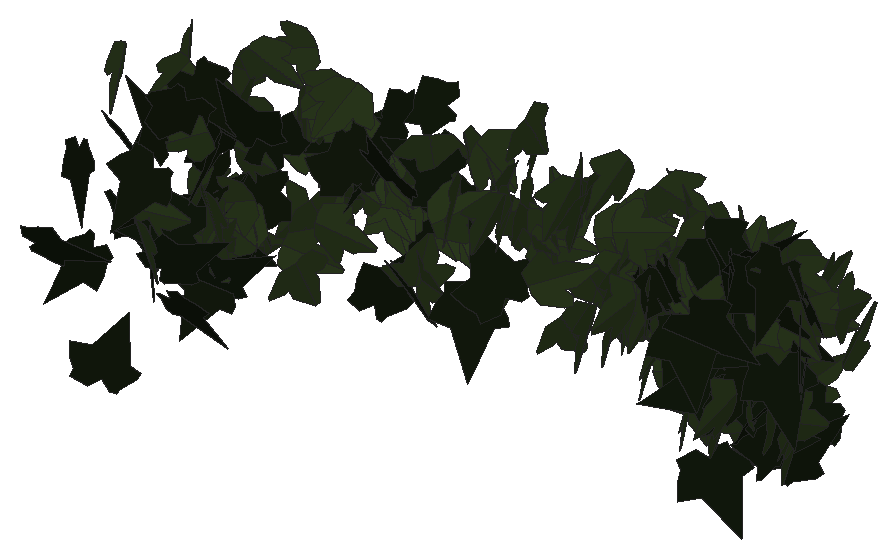
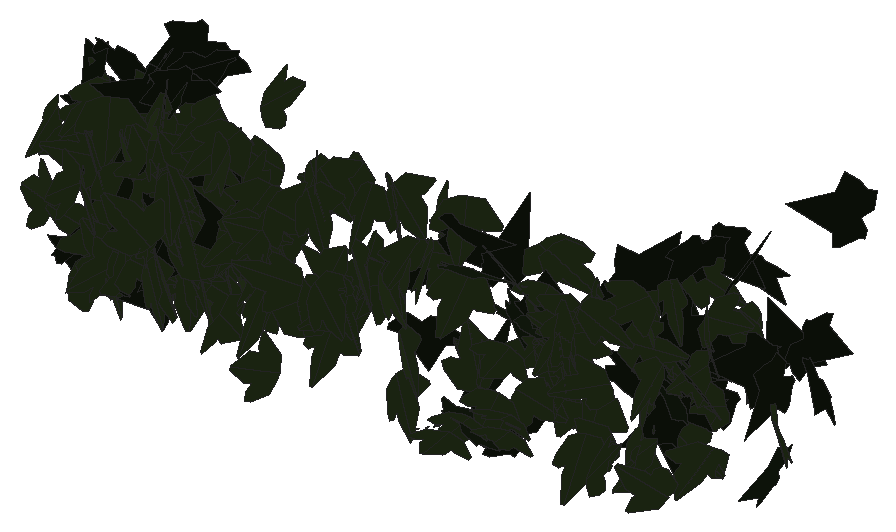
# SketchUp Ruby script. Lengths in inches.
U = 1.inch
M = Sketchup.active_model
def pt(a) = Geom::Point3d.new(a.map { |v| v * U })
def face(e, loops, mat)
  f = e.add_face(loops[0].map { |a| pt(a) })
  loops[1..].each { |l| e.add_face(l.map { |a| pt(a) }).erase! }
  f.material = f.back_material = mat if mat
  f
end
# faces: each face lists its corners as indices into pts; further lists are holes
def faces(e, pts, list, mat = nil) = list.each { |f| face(e, (f[0].is_a?(Array) ? f : [f]).map { |l| l.map { |i| pts[i] } }, mat) }
# xy, xz, yz: faces in a plane at the given z, y or x. An outline is a flat list of corners, or four numbers for a rectangle; further outlines are holes
def ring(l) = l.size == 4 ? [[l[0], l[1]], [l[2], l[1]], [l[2], l[3]], [l[0], l[3]]] : l.each_slice(2).to_a
def flat(e, list, mat, &to3) = list.each { |f| face(e, (f[0].is_a?(Array) ? f : [f]).map { |l| ring(l).map { |u, v| to3.(u, v) } }, mat) }
def xy(e, z, list, mat = nil) = flat(e, list, mat) { |x, y| [x, y, z] }
def xz(e, y, list, mat = nil) = flat(e, list, mat) { |x, z| [x, y, z] }
def yz(e, x, list, mat = nil) = flat(e, list, mat) { |y, z| [x, y, z] }
def lines(e, pts, list) = list.each { |a, b| e.add_line(pt(pts[a]), pt(pts[b])) }
# prism: a flat outline (further loops are holes) pulled along v
def prism(e, loops, v, mat = nil)
  f = face(e, loops, mat); d = Geom::Vector3d.new(v.map { |x| x * U })
  f.pushpull(f.normal.samedirection?(d) ? d.length : -d.length)
end
def box(e, o, s, mat = nil) = prism(e, [[o, [o[0] + s[0], o[1], o[2]], [o[0] + s[0], o[1] + s[1], o[2]], [o[0], o[1] + s[1], o[2]]]], [0, 0, s[2]], mat)
def at(x, y, z, deg = 0) = Geom::Transformation.translation(pt([x, y, z])) * Geom::Transformation.rotation(ORIGIN, Z_AXIS, deg.degrees)
def axes(o, x, y, z) = Geom::Transformation.new([*x, 0, *y, 0, *z, 0, *pt(o).to_a, 1])
def part(name) = M.definitions.add(name)
# library, detail: a bought-in or finely detailed component or shape, given as its bounding box
def library(name, o, s) = part(name).tap { |d| box(d.entities, o, s) }
def detail(e, o, s) = box(e.add_group.entities, o, s)
def put(e, d, t, mat = nil) = e.add_instance(d, t).tap { |i| i.material = mat if mat }
def group(e, t, mat = nil) = e.add_group.tap { |g| g.transformation = t; g.material = mat if mat }.entities
root = M.entities
M.materials.add("efeu1").color = [18, 25, 13]
M.materials.add("efeu2").color = [43, 57, 29]
c1 = part("ivyleaf_10")
p = [[0,0.5,-0.03],[-0.0625,2.02,-0.43],[-0.19,2.01,-0.46],[-0.54,1.05,-0.29],[-0.52,0.625,-0.18],[-0.83,0.76,-0.28],
  [-1.16,0.64,-0.33],[-1.15,0.33,-0.24],[-0.77,-0.39,0.02],[-0.3,-0.51,0.16],[0.04,-0.48,0.23],[-0.02,2.01,-0.4375],
  [-0.06,2.01,-0.43],[0.04,-0.49,0.23],[0.67,-0.49,0.14],[1.38,0.36,-0.2],[1.375,0.51,-0.24],[0.81,0.65,-0.19],
  [0.62,0.59,-0.15],[0.6,1.09,-0.28],[0.5,1.23,-0.31]]
faces(c1.entities,p,[[0,1,2,3,4,5,6,7,8,9,10],[11,12,0,13,14,15,16,17,18,19,20]],"efeu2")
c2 = part("ivyleaf_9")
p = [[1.54,2.16,1.25],[1.36,2.04,1.19],[-0.21,0.99,0.68],[-0.71,1.11,0.82],[-0.85,0.86,0.67],[-0.8,0.17,0.21],
  [-0.9,-0.01,0.1],[-0.67,-0.16,-0.02],[-0.08,-0.08,-0.05],[-0.03,-0.6,-0.4],[0.65,-0.88,-0.66],[0.83,-0.6,-0.49],
  [1.29,-0.42,-0.43],[1.8125,-0.07,-0.26],[1.21,0.44,0.15]]
faces(c2.entities,p,[[0,1,2,3,4,5,6,7,8,9,10,11,12,13,14]],"efeu1")
put(root,c1,axes([4.54,225.17,200.76],[0.36183,-0.29812,0.1738],[0.13554,-0.10881,-0.46882],[0.31735,0.38638,0.00207]))
put(root,c2,axes([5.6,222.72,200.27],[-0.24673,-0.00364,-0.38497],[0.39976,0.00318,-0.23762],[0.00499,-0.43497,0.00149]))
put(root,c2,axes([5.83,223.46,200.53],[0.43405,-0.05514,-0.16333],[-0.16537,0.03848,-0.42155],[0.07049,0.42977,0.01679]))
put(root,c2,axes([5.71,223.76,198.8125],[0.31945,-0.31871,0.01317],[0.01265,-0.0064,-0.45219],[0.34425,0.29599,0.0044]))
put(root,c1,axes([6.26,224.97,201.79],[0.26337,-0.21685,0.36553],[0.28954,-0.22325,-0.34106],[0.31112,0.39133,0.00798]))
put(root,c1,axes([6.8,224.12,201.73],[0.12917,0.19852,-0.38284],[-0.20895,-0.31318,-0.24103],[-0.40046,0.22745,0.00227]))
put(root,c1,axes([6.96,225.62,201.15],[-0.00251,0.23333,0.3818],[-0.1357,0.35112,-0.23291],[-0.44977,-0.10723,0.06814]))
put(root,c1,axes([7.12,223.98,198.74],[0.22464,0.36802,0.25317],[0.13154,0.21632,-0.43117],[-0.42689,0.26032,0.00037]))
put(root,c2,axes([7.32,220.92,199.6875],[-0.01481,-0.00344,-0.45216],[0.17246,-0.40463,-0.00191],[-0.43675,-0.15965,0.01458]))
put(root,c2,axes([7.18,222.16,199.75],[0.03567,0.31059,-0.31488],[-0.00014,0.30365,0.32394],[0.46844,-0.02356,0.02407]))
put(root,c1,axes([7.15,225.28,198.59],[0.23345,0.1331,-0.36738],[0.3326,0.17324,0.26387],[0.23577,-0.37616,-0.00847]))
put(root,c1,axes([7.77,223.61,198.62],[0.16189,-0.03722,-0.42292],[-0.3979,0.17451,-0.15785],[0.19022,0.39672,0.02975]))
put(root,c2,axes([7.67,222.5,201.38],[-0.03385,-0.40787,0.15384],[0.01139,0.14755,0.42544],[-0.46844,0.03306,-0.00077]))
put(root,c1,axes([7.85,224.05,201.81],[-0.37286,0.13555,0.23637],[-0.25083,0.02389,-0.38172],[-0.137,-0.41265,0.05555]))
put(root,c1,axes([7.69,223.375,200.01],[-0.01212,-0.03609,-0.45069],[0.13019,0.41625,-0.03929],[0.45124,-0.12106,-0.00077]))
put(root,c1,axes([8.11,224.7,201.01],[0.12938,0.06125,-0.43021],[-0.41855,-0.14541,-0.13912],[-0.16968,0.40538,0.01511]))
put(root,c2,axes([8.09,223.59,200.21],[-0.40829,0.21371,-0.02618],[0.02328,-0.01302,-0.45164],[-0.23123,-0.37866,0.00075]))
put(root,c2,axes([8.03,222.65,202.16],[0.03166,0.1171,-0.43463],[-0.07798,-0.41171,-0.12524],[-0.4622,0.07749,-0.00864]))
put(root,c1,axes([8.1875,222.82,201.5],[-0.18755,-0.05401,0.41096],[-0.35248,-0.22848,-0.18165],[0.24758,-0.3662,0.05272]))
put(root,c2,axes([7.87,223.53,201.07],[-0.01659,0.09814,-0.48999],[-0.16945,0.46011,0.09789],[0.47012,0.16931,0.01799]))
put(root,c1,axes([8.1875,224.66,198.61],[-0.26568,0.1929,-0.31458],[-0.27339,0.16657,0.32458],[0.27457,0.35252,0.01878]))
put(root,c2,axes([7.7,222.06,199.6875],[-0.06312,0.0246,-0.44757],[0.44742,-0.11679,-0.06546],[-0.12863,-0.41831,-0.00804]))
put(root,c1,axes([8.25,225.77,201.98],[0.19275,-0.05155,-0.40907],[-0.41552,0.08262,-0.19282],[0.10441,0.42396,-0.01216]))
put(root,c2,axes([8.27,222.5,199.64],[-0.19769,-0.07633,0.40265],[-0.3878,-0.14479,-0.20624],[0.17675,-0.40303,-0.00216]))
put(root,c2,axes([8.11,221.61,201.27],[-0.42989,-0.1683,-0.0516],[0.04917,0.01972,-0.44945],[0.18301,-0.40064,-0.00044]))
put(root,c1,axes([7.64,222.0625,200.12],[0.02616,-0.01223,-0.45152],[0.46101,-0.07957,0.0271],[-0.08656,-0.42749,0.00787]))
put(root,c2,axes([7.875,223.16,202.37],[0.06304,-0.27853,-0.34215],[-0.02745,0.32919,-0.29454],[0.46474,0.05723,0.02902]))
put(root,c1,axes([7.98,224.52,201.58],[0.20664,-0.34128,0.19772],[0.10219,-0.16491,-0.4069],[0.40935,0.21344,0.00177]))
put(root,c1,axes([8.01,221.49,200.04],[-0.32999,0.27319,-0.15156],[0.114,-0.10057,-0.42623],[-0.31437,-0.32323,0.00452]))
put(root,c2,axes([8.07,223.64,199.52],[-0.18935,0.3981,-0.00095],[-0.01202,-0.00391,0.45223],[0.42979,0.17528,0.01223]))
put(root,c1,axes([8.07,224.41,198.49],[-0.05405,-0.13447,-0.42708],[0.14284,0.38879,-0.14917],[0.44428,-0.14136,-0.004]))
put(root,c1,axes([7.88,224.97,202.06],[-0.27448,-0.04326,-0.36439],[0.37794,0.02611,-0.26734],[0.05033,-0.43205,0.02033]))
put(root,c1,axes([7.89,222.75,198.95],[0.10336,0.03509,0.4398],[0.39999,0.20468,-0.10484],[-0.22368,0.38223,0.01576]))
put(root,c2,axes([8.03,223.39,199.02],[0.022,0.04137,-0.44985],[0.08807,0.42497,0.04627],[0.46095,-0.08317,0.01263]))
put(root,c1,axes([8.3,223.41,199.67],[0.11664,0.30229,-0.30531],[-0.13236,-0.26742,-0.33327],[-0.43542,0.16227,0.01952]))
put(root,c2,axes([8.34,223.1,201.09],[-0.30799,0.18174,-0.28458],[0.2366,-0.16478,-0.35127],[-0.26434,-0.35923,0.01715]))
put(root,c2,axes([7.91,218.71,201],[0.29999,-0.0856,0.33659],[0.35326,-0.02016,-0.2975],[0.07699,0.42602,0.05355]))
put(root,c1,axes([8.31,223.07,198.58],[-0.40206,-0.2131,0.07515],[0.07243,0.02826,0.44602],[-0.23197,0.37817,0.00902]))
put(root,c2,axes([8.47,223.18,198.75],[0.08919,0.40301,-0.14704],[-0.03681,-0.13733,-0.4278],[-0.45979,0.08917,0.00572]))
put(root,c1,axes([8.27,225.63,198.73],[-0.09776,0.01057,0.49024],[0.21718,-0.44724,0.05295],[0.43963,0.2233,0.08285]))
put(root,c1,axes([8.7,223.46,200.05],[0.20038,-0.00751,-0.40911],[-0.41187,0.10355,-0.18912],[0.10453,0.42243,0.03909]))
put(root,c1,axes([8.66,223.64,199.21],[0.22842,0.15989,0.35865],[-0.30173,-0.20222,0.27571],[0.27838,-0.35038,0.00454]))
put(root,c1,axes([8.43,222.86,200.22],[-0.39131,0.23971,-0.02288],[0.01836,-0.01417,-0.45181],[-0.25932,-0.36272,0.00253]))
put(root,c1,axes([8.49,223.04,199.13],[-0.00135,0.18402,0.40992],[-0.13485,0.37742,-0.18367],[-0.45003,-0.11365,0.0538]))
put(root,c2,axes([8.45,222.92,198.64],[-0.21008,-0.37577,0.10497],[-0.05154,-0.08895,-0.44005],[0.41704,-0.20028,-0.00151]))
put(root,c1,axes([8.19,224.16,200.59],[0.00292,-0.01108,-0.45224],[0.40265,-0.22398,0.00835],[-0.24203,-0.37274,0.00843]))
put(root,c2,axes([8.91,224.15,200.01],[-0.14556,-0.11685,-0.41261],[-0.34535,-0.23521,0.18502],[-0.2833,0.34677,-0.01354]))
put(root,c2,axes([8.3,221.76,199.32],[0.06353,-0.03838,0.44646],[0.46287,0.05111,-0.05632],[-0.04931,0.43028,0.04651]))
put(root,c1,axes([8.42,224.12,199.07],[-0.15519,0.09457,0.4658],[0.38148,-0.26751,0.18141],[0.28353,0.4117,0.01088]))
put(root,c1,axes([8.67,225.52,199.03],[-0.16969,-0.41671,-0.21808],[0.10169,0.19385,-0.44953],[0.4592,-0.19691,0.01896]))
put(root,c2,axes([8.46,221.83,198.66],[0.46875,0.012,0.0275],[0.02857,0.00013,-0.45156],[-0.01294,0.43483,-0.00062]))
put(root,c2,axes([8.88,223.6,201.38],[0.25762,-0.06226,0.37273],[-0.37268,0.09686,0.25636],[-0.12429,-0.41948,0.00388]))
put(root,c2,axes([9.02,224.14,200.87],[0.05711,-0.00411,0.44902],[-0.46167,0.06077,0.05505],[-0.06568,-0.43071,0.00348]))
put(root,c1,axes([8.44,225.36,200.33],[0.11129,0.08107,0.43136],[0.35058,0.2582,-0.13635],[-0.29227,0.34057,0.0007]))
put(root,c2,axes([8.69,219.51,198.25],[-0.31326,-0.02588,0.33607],[0.34836,-0.0664,0.29557],[0.035,0.42912,0.066]))
put(root,c2,axes([8.48,222.84,198.6],[0.04105,-0.05266,0.44733],[0.46709,0.03157,-0.03573],[-0.02922,0.43065,0.05732]))
put(root,c1,axes([9,225.32,200.88],[-0.29157,-0.33694,0.05512],[0.02483,-0.08541,-0.44295],[0.36753,-0.26153,0.07365]))
put(root,c1,axes([9.06,225.34,201.02],[-0.14761,-0.41067,0.04531],[0.05403,-0.06202,-0.44475],[0.44272,-0.12935,0.06938]))
put(root,c1,axes([9.07,224.82,201.63],[-0.05659,0.40376,-0.15928],[0.01062,-0.15313,-0.42332],[-0.46626,-0.05249,0.00969]))
put(root,c1,axes([8.95,224.61,198.62],[0.13236,0.10625,0.41977],[0.26436,0.32243,-0.16557],[-0.36511,0.27198,0.0323]))
put(root,c1,axes([9.16,225.21,201.14],[-0.19867,-0.29512,-0.35134],[0.19885,0.28966,-0.35575],[0.41351,-0.28107,0.00227]))
put(root,c1,axes([9.39,225.23,200.85],[0.16987,-0.36292,-0.18827],[-0.07128,0.16868,-0.41132],[0.43218,0.17047,0.00616]))
put(root,c1,axes([9.25,225.14,200.99],[0.20536,-0.34321,0.19533],[0.11879,-0.15351,-0.40754],[0.40549,0.21879,0.02047]))
put(root,c1,axes([9.07,225.54,201.16],[-0.05815,-0.03764,0.44721],[0.46583,0.01224,0.05728],[-0.01821,0.4332,0.03724]))
put(root,c1,axes([9.35,224.97,201.33],[0.20443,0.23049,0.32932],[0.18373,0.2684,-0.30894],[-0.381,0.2531,0.02772]))
put(root,c2,axes([9.875,225,201.03],[-0.43882,0.1553,-0.00457],[-0.11474,-0.28672,-0.32178],[-0.12242,-0.28792,0.31797]))
put(root,c1,axes([9.83,224.69,202.12],[0.34076,0.02454,-0.36507],[-0.36493,-0.01348,-0.34153],[-0.0266,0.49922,0.00873]))
put(root,c1,axes([9.61,223.9,198.78],[-0.17962,-0.41604,-0.2113],[0.10172,0.18606,-0.45281],[0.4554,-0.20566,0.0178]))
put(root,c1,axes([9.86,225.28,200.59],[-0.39042,0.1553,0.19297],[-0.2573,-0.28672,-0.23315],[0.04565,-0.28792,0.33626]))
put(root,c1,axes([9.79,225.67,199.75],[-0.1791,-0.19339,0.3667],[-0.12879,-0.3406,-0.25261],[0.41478,-0.18926,0.0799]))
put(root,c1,axes([9.64,225.51,200.47],[0.36519,-0.21356,0.17794],[0.15645,-0.09105,-0.41593],[0.25074,0.36787,0.00035]))
put(root,c1,axes([9.52,225.24,199.61],[-0.22554,0.06303,0.44177],[0.42805,-0.10934,0.23414],[0.12612,0.48381,-0.00464]))
put(root,c1,axes([10.1,224.67,202.15],[0.36094,0.20865,-0.27602],[-0.24987,-0.11872,-0.4165],[-0.23934,0.4386,0.01857]))
put(root,c1,axes([9.64,224.72,199.31],[-0.08162,0.01517,-0.49306],[0.48478,-0.08999,-0.08302],[-0.09126,-0.4916,-0.00002]))
put(root,c1,axes([9.86,225.3,200.57],[-0.33479,-0.24256,-0.19259],[0.31096,-0.14498,-0.30376],[0.10923,-0.33071,0.27442]))
put(root,c1,axes([10,224.93,201.45],[-0.41218,-0.13322,-0.16711],[0.22482,-0.21842,-0.32587],[0.0165,-0.35181,0.2656]))
put(root,c1,axes([9.93,226.15,199.12],[-0.35211,-0.22187,-0.19092],[0.31078,-0.24033,-0.22941],[0.01197,-0.28677,0.33998]))
put(root,c1,axes([9.97,226.09,199.43],[-0.32329,-0.22187,-0.23346],[0.33916,-0.24033,-0.18848],[-0.03412,-0.28677,0.33858]))
put(root,c2,axes([10.15,225.47,201.03],[-0.32386,-0.26781,-0.17271],[0.31389,-0.14647,-0.30016],[0.13151,-0.30992,0.29111]))
put(root,c2,axes([10.36,224.46,200.64],[-0.43667,-0.13546,0.20241],[0.19803,0.04442,0.45696],[-0.14178,0.47925,0.01485]))
put(root,c1,axes([10.22,226.08,199.67],[-0.41368,-0.13062,-0.16591],[0.21662,-0.1581,-0.36622],[0.05158,-0.38362,0.20742]))
put(root,c2,axes([10.52,225.125,201.02],[-0.39629,0.22008,-0.21099],[0.18183,-0.10713,-0.45328],[-0.24472,-0.43599,0.00488]))
put(root,c1,axes([10.28,225.73,200.46],[-0.37867,-0.13062,-0.23075],[0.27769,-0.1581,-0.32577],[0.01449,-0.38362,0.21283]))
put(root,c2,axes([10.93,226.8,199.26],[-0.33749,0.16021,0.26699],[-0.31857,-0.24368,-0.21525],[0.07299,-0.32277,0.29504]))
put(root,c2,axes([11.02,224.99,201.76],[-0.41939,0.25191,0.1032],[-0.09382,0.04419,-0.48913],[-0.25556,-0.42964,0.0102]))
put(root,c2,axes([10.69,226.4,199.22],[-0.31081,-0.24024,-0.22948],[0.35203,-0.20051,-0.21509],[0.01351,-0.30217,0.32518]))
put(root,c1,axes([10.67,226.39,199.22],[-0.33547,-0.21588,-0.22338],[0.32344,-0.16093,-0.28221],[0.05962,-0.34165,0.27409]))
put(root,c2,axes([10.78,224.64,198.23],[-0.06533,-0.07929,0.48933],[0.40675,0.27355,0.09863],[-0.28335,0.41095,0.02876]))
put(root,c2,axes([11.35,225.8,201.87],[-0.42775,0.13023,0.12905],[-0.1868,-0.19329,-0.36318],[-0.05336,-0.36729,0.23688]))
put(root,c1,axes([10.87,226.71,198.99],[-0.33913,-0.24024,-0.18866],[0.32004,-0.20051,-0.2573],[0.05726,-0.30217,0.32073]))
put(root,c2,axes([11.42,224.25,201.08],[0.41089,-0.24765,0.14084],[-0.12088,0.07229,0.47975],[-0.25799,-0.4283,-0.00047]))
put(root,c1,axes([11.66,225.125,201.1],[-0.3355,-0.30829,-0.20591],[0.13858,0.15328,-0.4553],[0.34386,-0.36257,-0.01741]))
put(root,c1,axes([11.72,224.64,199.06],[-0.3476,-0.35437,0.05994],[0.04569,0.03914,0.49637],[-0.35649,0.35056,0.00517]))
put(root,c2,axes([11.75,224.53,198.71],[0.34576,-0.35884,0.04099],[-0.02732,0.0306,0.49831],[-0.36014,-0.34684,0.00155]))
put(root,c1,axes([11.78,224.61,198.99],[-0.13602,0.03513,0.47986],[0.46234,-0.12849,0.14046],[0.13318,0.48193,0.00247]))
put(root,c2,axes([12.53,224.46,201.51],[-0.32447,-0.16208,-0.34417],[-0.29405,-0.18014,0.36205],[-0.24136,0.43736,0.02159]))
put(root,c1,axes([12.26,224.34,202.05],[-0.4001,-0.29763,-0.03659],[0.0291,0.02219,-0.49866],[0.29846,-0.40115,-0.00043]))
put(root,c1,axes([12.27,225.4,201.55],[-0.22558,0.44361,-0.04823],[0.02101,-0.04343,-0.49767],[-0.44573,-0.22655,0.00095]))
put(root,c1,axes([12.66,225.36,201.57],[0.03301,0.4166,0.2745],[0.02881,0.27305,-0.41787],[-0.49808,0.04341,-0.00598]))
put(root,c1,axes([12.89,225.35,198.7],[0.02053,-0.49835,0.03495],[0.00001,-0.03498,-0.49877],[0.49958,0.02048,-0.00143]))
put(root,c1,axes([12.85,225.77,201.02],[0.16221,-0.4484,0.15042],[0.03839,-0.14601,-0.47666],[0.4714,0.16619,-0.01294]))
put(root,c1,axes([12.57,225.65,200.84],[0.01119,-0.09727,0.49032],[0.44175,-0.22762,-0.05524],[0.23396,0.43443,0.08084]))
put(root,c1,axes([12.94,225.16,199.46],[0.21035,-0.45358,0.00422],[0.00131,-0.00404,-0.49998],[0.4536,0.21036,-0.00052]))
put(root,c1,axes([12.74,224.09,200.88],[0.10913,0.09599,-0.47841],[0.36179,0.31303,0.14534],[0.32742,-0.37789,-0.00113]))
put(root,c1,axes([13.07,226.33,201.63],[0.27369,-0.41576,0.04728],[0.02489,-0.04022,-0.49776],[0.4177,0.27481,-0.00132]))
put(root,c1,axes([13.03,224.01,201.51],[0.20062,-0.24316,0.38811],[0.25246,-0.2948,-0.3152],[0.38212,0.32244,0.0045]))
put(root,c2,axes([13.33,224.19,199.34],[-0.32301,-0.2957,-0.2413],[0.17982,0.16092,-0.43791],[0.33664,-0.36969,0.00239]))
put(root,c1,axes([13.5,225.48,202.38],[-0.02546,-0.41841,-0.27255],[0.08153,0.26576,-0.4156],[0.49265,-0.06561,0.05469]))
put(root,c1,axes([13.66,225.1875,200.64],[-0.46285,-0.08614,-0.16837],[0.16493,0.034,-0.47079],[0.09256,-0.49135,-0.00306]))
put(root,c1,axes([13.76,225,201.07],[0.10083,-0.33579,-0.35648],[0.02489,0.367,-0.33866],[0.48909,0.05055,0.09072]))
put(root,c1,axes([13.42,225.26,200.5625],[-0.2114,0.05809,-0.44937],[0.43712,-0.10441,-0.21914],[-0.11929,-0.48551,-0.00664]))
put(root,c1,axes([14,225.52,200.09],[0.18502,-0.19871,-0.41986],[-0.27498,0.31739,-0.27139],[0.37437,0.33133,0.00816]))
put(root,c1,axes([13.95,226.24,200.61],[0.00616,-0.46596,0.18124],[0.00706,-0.18115,-0.46598],[0.49991,0.00831,0.00435]))
put(root,c1,axes([13.99,223.98,201.6],[-0.06315,-0.44931,0.21008],[-0.02556,-0.20854,-0.45371],[0.49534,-0.06804,0.00337]))
put(root,c2,axes([14.19,223.93,199.88],[-0.4377,-0.24044,0.02459],[0.03204,-0.0073,0.49892],[-0.23957,0.43833,0.0218]))
put(root,c1,axes([13.85,225.52,200.13],[-0.0493,-0.19347,-0.45841],[0.35656,0.30756,-0.16815],[0.34704,-0.34348,0.10764]))
put(root,c1,axes([14.26,223.9,201.62],[0.22569,-0.35252,-0.27348],[-0.14742,0.23034,-0.41858],[0.4211,0.26958,0.00003]))
put(root,c1,axes([14.27,225.64,200.59],[0.44303,0.01856,0.23103],[-0.23084,-0.00944,0.44342],[0.02083,-0.49957,0.0002]))
put(root,c1,axes([14.72,225,199.05],[-0.15714,-0.40235,-0.25184],[0.09168,0.23456,-0.43195],[0.46573,-0.18193,0.00005]))
put(root,c1,axes([14.91,225.32,201.71],[-0.03174,-0.49526,0.06088],[-0.00834,-0.06047,-0.49626],[0.49892,-0.03252,-0.00442]))
put(root,c1,axes([14.99,224.77,201.91],[-0.07742,-0.431,0.24134],[0.00157,-0.2445,-0.43614],[0.49397,-0.06677,0.03921]))
put(root,c1,axes([14.94,225.57,199.42],[-0.45616,-0.14963,0.13976],[0.13432,0.03889,0.48005],[-0.15453,0.4755,0.00472]))
put(root,c1,axes([15.1,226.05,201.78],[-0.05619,-0.29947,0.39643],[0.05616,-0.40023,-0.29438],[0.49365,0.01145,0.07861]))
put(root,c1,axes([14.85,225.24,201.97],[0.19859,-0.17373,0.42471],[0.35283,-0.23808,-0.26236],[0.29339,0.4039,0.02803]))
put(root,c1,axes([15.21,226.21,198.59],[0.07536,-0.24821,0.42745],[-0.05472,0.42554,0.25675],[-0.49125,-0.08548,0.03697]))
put(root,c1,axes([14.93,226.02,200.42],[0.09677,0.03183,-0.48951],[0.48115,0.09104,0.10103],[0.09556,-0.49061,-0.01301]))
put(root,c1,axes([15.37,224.65,201.81],[0.09142,-0.49127,0.01732],[0.00197,-0.01725,-0.4997],[0.49157,0.09143,-0.00122]))
put(root,c1,axes([15.38,224.89,199.43],[0.16765,-0.42147,0.21038],[0.10834,-0.18282,-0.45259],[0.45843,0.19734,0.03002]))
put(root,c1,axes([15.73,225.73,199.55],[-0.01661,-0.35368,-0.35303],[0.07082,0.348,-0.35197],[0.49468,-0.0617,0.03853]))
put(root,c1,axes([15.56,223.33,200.85],[-0.11444,-0.14607,0.46429],[0.28141,0.3693,0.18554],[-0.39713,0.30378,-0.00231]))
put(root,c1,axes([15.7,225.41,199.72],[-0.16275,0.37287,-0.29065],[0.08468,-0.27943,-0.40589],[-0.46513,-0.18134,0.0278]))
put(root,c1,axes([15.99,225.48,200.06],[-0.05101,0.44536,-0.22149],[0.02075,-0.22055,-0.44825],[-0.49696,-0.05492,0.00402]))
put(root,c1,axes([15.94,225.38,200.78],[0.1932,0.18459,-0.42261],[0.21694,0.36795,0.2599],[0.40695,-0.28379,0.06209]))
put(root,c1,axes([16.06,224.79,199.84],[0.17202,-0.42027,0.20925],[0.11159,-0.17987,-0.45298],[0.45603,0.20254,0.03191]))
put(root,c1,axes([15.97,225.38,201.55],[0.17306,0.37407,0.28306],[0.12014,0.2563,-0.41216],[-0.45345,0.21067,-0.00117]))
put(root,c1,axes([16.14,224.79,200.65],[0.13643,-0.4385,0.19775],[0.0687,-0.18568,-0.45913],[0.4761,0.15245,0.00959]))
put(root,c1,axes([16.08,225.61,200.89],[-0.18805,-0.21071,-0.4126],[0.28284,0.30047,-0.28235],[0.36693,-0.33959,0.00619]))
put(root,c1,axes([16.22,226.21,199.33],[0.06035,0.38528,-0.31292],[-0.05672,-0.3078,-0.38992],[-0.49309,0.08256,0.00655]))
put(root,c1,axes([15.93,224.65,200.66],[-0.22471,0.04426,-0.44446],[0.44099,-0.05702,-0.22864],[-0.07092,-0.49476,-0.01341]))
put(root,c1,axes([16.61,225.36,200.65],[0.13241,0.04,-0.48049],[-0.45541,-0.15325,-0.13826],[-0.15833,0.47425,-0.00415]))
put(root,c1,axes([16.375,225.2,201.41],[0.0531,-0.15512,0.47235],[0.17661,-0.43817,-0.16375],[0.46475,0.18423,0.00826]))
put(root,c1,axes([16.61,225.28,200.57],[0.06446,-0.25093,-0.42765],[0.02147,0.43225,-0.25039],[0.49536,0.01391,0.0665]))
put(root,c1,axes([16.61,225,200.55],[-0.07009,0.3811,0.316],[-0.05376,0.3114,-0.38748],[-0.49214,-0.08829,-0.00267]))
put(root,c1,axes([16.76,224.99,200.2],[0.00701,-0.40506,0.29306],[0.04343,-0.29148,-0.40392],[0.49806,0.03111,0.0311]))
put(root,c1,axes([16.66,225.6875,202.21],[-0.35559,0.29806,-0.18633],[0.14648,-0.11528,-0.46395],[-0.31953,-0.38454,-0.00534]))
put(root,c1,axes([16.43,224.62,201.64],[0.13571,-0.07548,-0.47527],[0.4761,-0.05086,0.14402],[-0.07008,-0.49165,0.05807]))
put(root,c1,axes([16.69,224.78,199.91],[-0.36254,-0.05728,-0.33953],[0.33498,0.05544,-0.36704],[0.07969,-0.49361,-0.00183]))
put(root,c1,axes([16.92,225.71,198.85],[0.3912,-0.27709,0.14208],[-0.11094,0.08914,0.47932],[-0.29096,-0.40654,0.00826]))
put(root,c1,axes([16.89,224.83,199.45],[0.25108,-0.37271,0.2192],[0.11569,-0.18632,-0.44933],[0.41662,0.27635,-0.00732]))
put(root,c1,axes([16.8125,225.3125,202.3125],[-0.29222,-0.18317,-0.36201],[0.3096,0.18766,-0.34487],[0.26221,-0.42571,0.00374]))
put(root,c2,axes([16.74,225.03,200.51],[0.40277,0.23029,-0.18639],[0.15554,0.10337,0.46381],[0.25216,-0.4316,0.01163]))
put(root,c1,axes([16.98,224.62,200.8],[0.2361,-0.29073,0.33126],[0.24323,-0.22744,-0.37298],[0.36756,0.33726,0.03403]))
put(root,c1,axes([16.89,225.22,199.625],[-0.05443,0.05251,0.49425],[0.42289,-0.25636,0.07381],[0.26116,0.42605,-0.0165]))
put(root,c1,axes([16.89,224.65,200.48],[-0.13136,-0.03193,0.48138],[0.45686,-0.16853,0.11349],[0.15501,0.46966,0.07345]))
put(root,c1,axes([16.97,226.76,199.58],[0.24119,-0.24227,-0.36487],[0.25074,-0.26514,0.3418],[-0.3591,-0.34786,-0.0064]))
put(root,c1,axes([17.57,225.05,200.36],[0.34089,0.11073,-0.34861],[-0.33158,-0.10764,-0.35843],[-0.15443,0.47556,0.00005]))
put(root,c1,axes([17.52,225.9375,201.55],[0.33006,-0.2988,-0.22755],[-0.16968,0.15162,-0.44522],[0.33507,0.37112,-0.00131]))
put(root,c1,axes([17.02,225.14,200.71],[0.06224,-0.00401,-0.49609],[0.48255,-0.11561,0.06147],[-0.1152,-0.48643,-0.01053]))
put(root,c1,axes([17.35,224.61,199.97],[0.09102,-0.26029,0.41709],[0.13086,-0.39605,-0.27571],[0.47391,0.15936,-0.00398]))
put(root,c1,axes([17.04,224.98,198.91],[0.10624,-0.02009,-0.48817],[0.4795,-0.0916,0.10812],[-0.09377,-0.49113,-0.00019]))
put(root,c2,axes([17.59,224.85,200.1875],[-0.42139,-0.15317,-0.2213],[0.21059,0.06836,-0.44831],[0.16759,-0.47103,0.0069]))
put(root,c2,axes([17.42,224.54,201.18],[0.00827,-0.25963,-0.42723],[0.02565,0.42695,-0.25896],[0.49927,-0.01763,0.02037]))
put(root,c1,axes([17.5,225.29,199.54],[-0.45235,-0.13977,0.16076],[0.15779,0.03367,0.47325],[-0.14312,0.47888,0.01365]))
put(root,c1,axes([17.35,224.64,200.625],[-0.03472,-0.04879,0.4964],[0.45543,0.19982,0.05149],[-0.20341,0.45573,0.03057]))
put(root,c2,axes([17.51,224.43,201.3125],[0.39613,-0.28637,-0.10522],[-0.07749,0.07234,-0.48863],[0.29509,0.40343,0.01293]))
put(root,c1,axes([17.81,225.71,201.18],[-0.00311,-0.48968,-0.10104],[-0.00581,0.10107,-0.48964],[0.49996,-0.00187,-0.00632]))
put(root,c1,axes([17.72,226.65,200.66],[-0.24329,-0.32598,0.29077],[0.17582,0.2316,0.40676],[-0.39988,0.30016,0.00194]))
put(root,c1,axes([17.67,224.8125,198.61],[0.16906,-0.16323,0.44133],[0.30345,-0.3206,-0.23481],[0.35964,0.34724,-0.00933]))
put(root,c1,axes([18.23,224.71,198.81],[-0.10481,0.1234,-0.47306],[-0.37079,0.29526,0.15917],[0.31864,0.38418,0.02962]))
put(root,c1,axes([17.82,225.02,200.37],[0.26991,0.40119,0.12725],[0.06601,0.10894,-0.4835],[-0.41568,0.27781,0.00584]))
put(root,c1,axes([17.9,222.71,201.53],[-0.03526,-0.02073,0.49832],[0.14406,-0.4787,-0.00972],[0.4775,0.1429,0.03973]))
put(root,c1,axes([17.89,224.41,202],[-0.06759,-0.16819,-0.46599],[0.16065,0.43745,-0.18119],[0.46864,-0.17422,-0.00509]))
put(root,c1,axes([17.86,225.54,199.88],[0.43375,-0.24517,-0.04182],[0.04238,-0.00999,0.4981],[-0.24508,-0.43565,0.01211]))
put(root,c1,axes([17.89,224.98,201.1875],[-0.0856,-0.41959,0.2581],[0.05026,0.25317,0.42823],[-0.49005,0.09926,-0.00116]))
put(root,c1,axes([18.05,225.92,199.4],[0.13054,-0.48248,0.01294],[0.0034,-0.01249,-0.49983],[0.48265,0.13059,0.00002]))
put(root,c2,axes([17.62,224.64,200.09],[0.22525,-0.16647,0.41418],[0.32175,-0.26102,-0.2799],[0.30941,0.39262,-0.01047]))
put(root,c1,axes([18.16,225.89,200.35],[0.0581,-0.0134,-0.49643],[-0.1308,0.48176,-0.02831],[0.47908,0.13315,0.05247]))
put(root,c1,axes([18.19,224.66,198.82],[-0.40431,-0.29384,0.01386],[-0.00808,-0.01246,-0.49978],[0.29405,-0.40436,0.00532]))
put(root,c2,axes([18.1,224.67,199.63],[-0.03196,0.07292,-0.49362],[-0.15562,0.4685,0.07928],[0.47409,0.15871,-0.00726]))
put(root,c1,axes([18.26,224.69,200.64],[-0.42233,-0.25434,0.08332],[-0.07041,-0.0446,-0.49301],[0.25822,-0.42816,0.00185]))
put(root,c1,axes([18.29,224.57,200.8],[0.22793,0.4088,0.17588],[-0.09462,-0.14857,0.46795],[0.43485,-0.2466,0.00964]))
put(root,c1,axes([18.02,224.47,201.08],[0.08313,-0.00422,-0.49302],[0.49262,0.0214,0.08288],[0.0204,-0.49952,0.00771]))
put(root,c1,axes([18.67,225.26,201.62],[-0.11031,0.2195,-0.43549],[-0.24732,0.35964,0.24391],[0.42031,0.26922,0.02923]))
put(root,c1,axes([18.74,225.77,199.44],[-0.15938,-0.18205,0.43756],[-0.22028,-0.38028,-0.23846],[0.41961,-0.26878,0.04101]))
put(root,c2,axes([18.81,224.21,199.54],[-0.0736,-0.15274,-0.47038],[-0.19694,-0.42717,0.16952],[-0.45365,0.21022,0.00272]))
put(root,c2,axes([18.29,224.62,199.76],[-0.09943,-0.14254,0.46882],[0.25892,-0.42143,-0.07322],[0.41602,0.22822,0.15762]))
put(root,c1,axes([18.61,224.64,198.77],[0.14077,-0.47587,0.06107],[0.01448,-0.05941,-0.49625],[0.47956,0.14148,-0.00295]))
put(root,c1,axes([18.49,225.3125,201.27],[0.29394,0.33907,-0.22052],[0.14635,0.16497,0.44874],[0.37707,-0.32835,-0.00226]))
put(root,c2,axes([18.4,224.68,199.43],[0.03874,-0.0425,-0.49668],[0.07392,0.49316,-0.03643],[0.49299,-0.07061,0.04449]))
put(root,c2,axes([18.36,225.5,198.91],[-0.04362,-0.11313,-0.48508],[0.46435,0.16694,-0.08069],[0.18021,-0.45753,0.0905]))
put(root,c1,axes([18.75,224.95,201.28],[-0.29313,-0.38352,-0.13035],[-0.08144,-0.10182,0.4827],[-0.39679,0.30422,-0.00277]))
put(root,c1,axes([18.45,224.26,201.53],[0.16891,0.04804,-0.46815],[0.37797,0.28248,0.16536],[0.28038,-0.40975,0.05911]))
put(root,c1,axes([18.8,225.64,198.99],[0.10096,0.4676,-0.14545],[0.02986,0.14235,0.47838],[0.48879,-0.10528,0.00082]))
put(root,c2,axes([18.5625,224.23,202.375],[0.09902,-0.17473,-0.45789],[0.11465,0.46244,-0.15167],[0.4765,-0.07496,0.13165]))
put(root,c1,axes([18.59,224.85,198.73],[0.04762,-0.08575,-0.49029],[0.38105,-0.31058,0.09133],[-0.32021,-0.38234,0.03577]))
put(root,c1,axes([19.25,224.7,198.83],[-0.10011,-0.08361,0.48269],[-0.37805,-0.30012,-0.1304],[0.31154,-0.39107,-0.00313]))
put(root,c1,axes([18.86,224.77,200.84],[-0.13266,0.27003,0.39936],[0.18219,-0.3554,0.30083],[0.44633,0.22533,-0.0041]))
put(root,c2,axes([19.12,224.18,201.87],[0.1445,-0.04906,-0.47614],[-0.44357,0.17322,-0.15246],[0.17991,0.46646,0.00654]))
put(root,c1,axes([19.08,225.45,200.84],[-0.41173,-0.27755,0.05869],[-0.04877,-0.03266,-0.49654],[0.27946,-0.41461,-0.00018]))
put(root,c1,axes([19.02,224.81,200.61],[-0.36246,0.32631,0.11021],[0.07865,-0.07736,0.48768],[0.33532,0.37086,0.00475]))
put(root,c1,axes([18.77,225.18,199.95],[0.38039,-0.20826,-0.24886],[0.22626,-0.10466,0.43342],[-0.23262,-0.44235,0.01462]))
put(root,c2,axes([18.8,224.6,201.77],[0.00365,-0.29895,0.40077],[0.11081,-0.39033,-0.29217],[0.48755,0.09095,0.0634]))
put(root,c1,axes([18.97,224.55,199.4375],[-0.10838,-0.2843,-0.39677],[0.17888,0.35502,-0.30325],[0.45416,-0.20768,0.02476]))
put(root,c2,axes([19.49,224.01,199.71],[-0.42966,0.00414,-0.25569],[-0.25569,0.00164,0.42968],[0.0044,0.49998,0.00071]))
put(root,c2,axes([19.07,224.49,199.78],[0.00581,-0.04421,-0.49801],[-0.08567,0.49059,-0.04455],[0.49257,0.08585,-0.00187]))
put(root,c1,axes([19.22,224.68,198.96],[-0.34594,0.35693,0.05407],[0.03419,-0.04216,0.49705],[0.35938,0.3476,0.00476]))
put(root,c1,axes([19.14,225.25,201.4],[0.24073,-0.41249,0.14798],[0.07451,-0.12785,-0.4776],[0.43185,0.252,-0.00008]))
put(root,c2,axes([18.83,225.48,200.96],[0.20141,-0.29688,0.34828],[0.21106,-0.27737,-0.3585],[0.40606,0.29142,0.01359]))
put(root,c2,axes([19.02,224.4,201.82],[0.06032,0.44703,-0.21571],[0.02915,0.21373,0.45108],[0.49549,-0.06699,-0.00027]))
put(root,c1,axes([19.33,224.96,199.6875],[0.17778,-0.44383,-0.14631],[-0.05592,0.13522,-0.47811],[0.46397,0.18636,-0.00156]))
put(root,c2,axes([19.18,224.54,199.58],[-0.03351,-0.39992,-0.29824],[0.05925,0.2936,-0.40036],[0.49534,-0.06217,0.02772]))
put(root,c1,axes([19.54,224.78,200.3125],[0.32825,0.21243,0.31164],[-0.26388,-0.16583,0.39098],[0.26947,-0.42116,0.00325]))
put(root,c2,axes([19.18,224.68,198.53],[0.09293,0.48748,0.06106],[-0.02343,-0.05767,0.49611],[0.49073,-0.09506,0.01213]))
put(root,c1,axes([19.35,225.54,198.95],[0.00193,0.00628,0.49996],[-0.05735,0.49666,-0.00602],[-0.4967,-0.05733,0.00264]))
put(root,c1,axes([19.64,225.15,201.07],[0.02116,0.07223,0.4943],[-0.27675,-0.41019,0.07179],[0.41589,-0.27663,0.02262]))
put(root,c1,axes([19.46,225.375,201.98],[-0.37699,-0.32735,-0.02692],[0.0207,0.01722,-0.49927],[0.3278,-0.37756,0.00057]))
put(root,c1,axes([19.58,226.28,200.85],[0.07025,-0.13207,0.4771],[-0.19966,0.43339,0.14937],[-0.45299,-0.2115,0.00815]))
put(root,c1,axes([19.43,225.39,199.03],[-0.05585,-0.45102,0.20847],[0.02692,0.20673,0.45446],[-0.49614,0.06199,0.00119]))
put(root,c1,axes([19.28,225.15,198.6],[-0.29929,-0.11892,0.38247],[0.35165,0.15056,0.32198],[-0.19175,0.46172,-0.00648]))
put(root,c1,axes([19.58,225.19,198.74],[0.20255,-0.4569,0.01464],[0.00575,-0.01346,-0.49979],[0.4571,0.20264,-0.0002]))
put(root,c1,axes([19.61,225.69,201.5],[0.31991,-0.38205,-0.04116],[-0.02429,0.03334,-0.4983],[0.38349,0.32082,0.00277]))
put(root,c2,axes([19.77,224.39,200.85],[-0.24728,-0.26878,0.34148],[-0.228,-0.25423,-0.36521],[0.36996,-0.33634,0.00317]))
put(root,c1,axes([19.57,223.47,199.79],[0.01252,-0.08425,0.49269],[0.15434,-0.46811,-0.08397],[0.47542,0.15419,0.01429]))
put(root,c1,axes([19.6,225.91,200.63],[0.37114,-0.32438,0.08386],[0.06377,-0.05447,-0.49292],[0.32892,0.37658,0.00094]))
put(root,c2,axes([19.59,222.47,201.71],[-0.19242,-0.40246,-0.22583],[0.10491,0.20012,-0.44603],[0.44941,-0.21904,0.00743]))
put(root,c2,axes([19.55,224.29,201.89],[0.22661,-0.22977,-0.38191],[0.25416,-0.28534,0.32247],[-0.36613,-0.34028,-0.01252]))
put(root,c1,axes([19.4375,224.2,201.61],[0.05749,0.00382,0.49667],[0.48188,0.12075,-0.05671],[-0.12038,0.48519,0.01021]))
put(root,c1,axes([19.95,225.52,198.49],[-0.06208,-0.15705,0.47062],[0.03064,-0.4746,-0.15433],[0.49518,0.00968,0.06855]))
put(root,c2,axes([19.66,222.42,202.01],[-0.00184,-0.05627,-0.49682],[0.22198,0.44509,-0.05123],[0.44802,-0.22075,0.02334]))
put(root,c2,axes([20.3,224.05,198.96],[-0.3375,0.28906,0.22921],[-0.17326,0.15007,-0.44436],[-0.32569,-0.37937,-0.00113]))
put(root,c1,axes([19.86,224.98,198.93],[0.39611,-0.25764,0.16346],[0.13676,-0.08953,-0.47253],[0.27275,0.41906,-0.00046]))
put(root,c1,axes([19.84,225.32,199.37],[-0.15428,-0.28778,0.37865],[0.17633,0.3351,0.32652],[-0.44171,0.23429,-0.00191]))
put(root,c1,axes([19.76,225.32,200.92],[0.06004,0.01319,-0.49621],[0.47884,0.13015,0.0614],[0.13079,-0.48258,0.003]))
put(root,c1,axes([19.97,224.86,201.88],[-0.23119,-0.24818,-0.36736],[0.2848,0.23439,-0.33757],[0.33977,-0.36534,0.03298]))
put(root,c2,axes([20.2,224.23,202.4],[-0.4293,-0.1306,-0.22055],[0.21058,0.06558,-0.44873],[0.14613,-0.47817,-0.0013]))
put(root,c2,axes([20.2,225.42,199.14],[-0.19424,-0.39569,0.23602],[-0.10591,-0.21093,-0.44078],[0.44839,-0.22122,-0.00187]))
put(root,c1,axes([20.1,224.26,199.25],[0.04995,-0.3665,-0.33643],[0.04366,-0.33359,0.36988],[-0.49558,-0.06633,-0.00133]))
put(root,c2,axes([20,224.59,198.19],[-0.03508,-0.03847,0.49728],[0.46998,0.16437,0.04587],[-0.16701,0.47064,0.02463]))
put(root,c2,axes([20.11,222.4,199.25],[-0.03115,-0.38829,-0.31347],[0.0535,0.30967,-0.3889],[0.49615,-0.05777,0.02225]))
put(root,c1,axes([20.32,224.52,198.96],[0.18254,-0.46101,0.0644],[0.02034,-0.06121,-0.49582],[0.46504,0.18363,-0.00359]))
put(root,c1,axes([20.05,224.125,200.86],[-0.11879,-0.05611,-0.48243],[0.45237,0.16799,-0.13093],[0.17678,-0.46758,0.01085]))
put(root,c2,axes([20.56,224.41,199.99],[0.00184,0.00203,0.49999],[0.00336,0.49998,-0.00204],[-0.49999,0.00337,0.00183]))
put(root,c1,axes([20.5,225.87,200.04],[0.16301,-0.32163,0.34638],[-0.13474,0.31958,0.36016],[-0.45307,-0.21076,0.01751]))
put(root,c2,axes([20.09,224.25,201.18],[0.21465,0.0079,-0.45151],[0.41417,0.19578,0.20032],[0.17996,-0.46001,0.07751]))
put(root,c1,axes([20.49,224.2,199.41],[-0.03097,-0.23901,-0.43808],[0.13349,0.41896,-0.23802],[0.48086,-0.1317,0.03786]))
put(root,c1,axes([20.39,224.8,201.2],[-0.1462,-0.16967,-0.44703],[0.28771,0.34215,-0.22396],[0.3819,-0.32272,-0.00241]))
put(root,c2,axes([20.38,224.48,201.46],[-0.11733,0.02813,-0.48522],[0.47231,-0.11118,-0.12066],[-0.11468,-0.48667,-0.00049]))
put(root,c2,axes([20.54,223.77,200.6875],[-0.04692,-0.45209,-0.20835],[0.02041,0.20735,-0.45452],[0.49738,-0.05115,-0.00101]))
put(root,c2,axes([20.42,224.58,201.87],[0.29026,-0.11456,-0.39067],[0.36748,-0.13279,0.31197],[-0.17523,-0.46823,0.00711]))
put(root,c1,axes([20.375,224.24,201.5],[0.21883,-0.00929,0.44948],[0.44957,0.00578,-0.21875],[-0.00113,0.49988,0.01088]))
put(root,c1,axes([20.79,225.26,201.36],[0.05026,-0.15832,-0.4716],[0.02653,0.47418,-0.15636],[0.49676,-0.00931,0.05607]))
